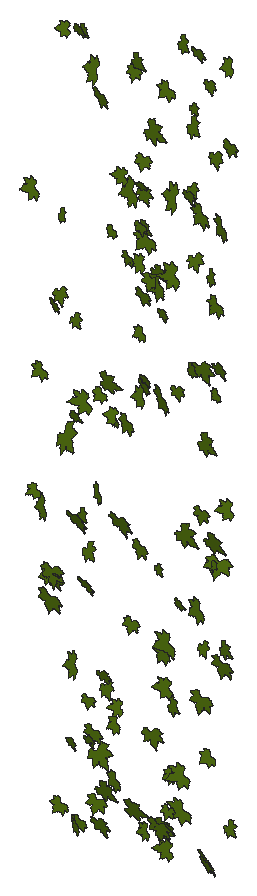
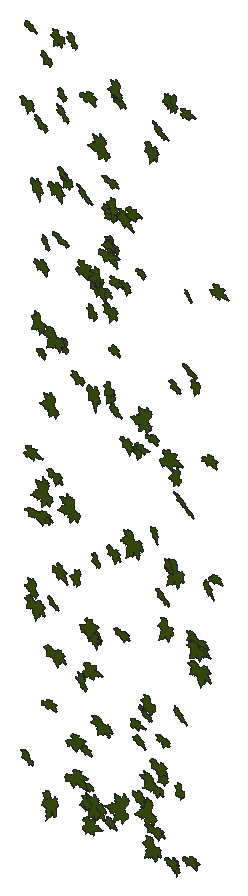
# SketchUp Ruby script. Lengths in inches.
U = 1.inch
M = Sketchup.active_model
def pt(a) = Geom::Point3d.new(a.map { |v| v * U })
def face(e, loops, mat)
  f = e.add_face(loops[0].map { |a| pt(a) })
  loops[1..].each { |l| e.add_face(l.map { |a| pt(a) }).erase! }
  f.material = f.back_material = mat if mat
  f
end
# faces: each face lists its corners as indices into pts; further lists are holes
def faces(e, pts, list, mat = nil) = list.each { |f| face(e, (f[0].is_a?(Array) ? f : [f]).map { |l| l.map { |i| pts[i] } }, mat) }
# xy, xz, yz: faces in a plane at the given z, y or x. An outline is a flat list of corners, or four numbers for a rectangle; further outlines are holes
def ring(l) = l.size == 4 ? [[l[0], l[1]], [l[2], l[1]], [l[2], l[3]], [l[0], l[3]]] : l.each_slice(2).to_a
def flat(e, list, mat, &to3) = list.each { |f| face(e, (f[0].is_a?(Array) ? f : [f]).map { |l| ring(l).map { |u, v| to3.(u, v) } }, mat) }
def xy(e, z, list, mat = nil) = flat(e, list, mat) { |x, y| [x, y, z] }
def xz(e, y, list, mat = nil) = flat(e, list, mat) { |x, z| [x, y, z] }
def yz(e, x, list, mat = nil) = flat(e, list, mat) { |y, z| [x, y, z] }
def lines(e, pts, list) = list.each { |a, b| e.add_line(pt(pts[a]), pt(pts[b])) }
# prism: a flat outline (further loops are holes) pulled along v
def prism(e, loops, v, mat = nil)
  f = face(e, loops, mat); d = Geom::Vector3d.new(v.map { |x| x * U })
  f.pushpull(f.normal.samedirection?(d) ? d.length : -d.length)
end
def box(e, o, s, mat = nil) = prism(e, [[o, [o[0] + s[0], o[1], o[2]], [o[0] + s[0], o[1] + s[1], o[2]], [o[0], o[1] + s[1], o[2]]]], [0, 0, s[2]], mat)
def at(x, y, z, deg = 0) = Geom::Transformation.translation(pt([x, y, z])) * Geom::Transformation.rotation(ORIGIN, Z_AXIS, deg.degrees)
def axes(o, x, y, z) = Geom::Transformation.new([*x, 0, *y, 0, *z, 0, *pt(o).to_a, 1])
def part(name) = M.definitions.add(name)
# library, detail: a bought-in or finely detailed component or shape, given as its bounding box
def library(name, o, s) = part(name).tap { |d| box(d.entities, o, s) }
def detail(e, o, s) = box(e.add_group.entities, o, s)
def put(e, d, t, mat = nil) = e.add_instance(d, t).tap { |i| i.material = mat if mat }
def group(e, t, mat = nil) = e.add_group.tap { |g| g.transformation = t; g.material = mat if mat }.entities
root = M.entities
M.materials.add("[Vegetation Blur 03]").color = [83, 114, 18]
c1 = part("ivy")
xy(c1.entities,0,[[0.782,0,0.786,0,0.787,0.005,0.789,0.009,0.821,0.072,0.875,0.147,1.001,0.272,1.073,0.331,1.137,0.363,1.178,0.379,1.223,0.384,1.272,0.383,1.311,0.374,1.36,0.355,1.399,0.334,1.491,0.285,1.541,0.244,1.583,0.199,1.617,0.15,1.64,0.128,1.662,0.115,1.717,0.105,1.745,0.093,1.784,0.054,1.819,0.057,1.854,0.064,1.882,0.075,1.896,0.074,1.91,0.071,1.937,0.063,1.964,0.053,1.99,0.038,2.016,0.015,2.034,0.002,2.04,0,2.038,0.003,2.036,0.007,2.033,0.038,2.036,0.068,2.045,0.1,2.055,0.116,2.064,0.123,2.077,0.129,2.088,0.129,2.106,0.132,2.118,0.13,2.179,0.132,2.207,0.133,2.225,0.133,2.242,0.138,2.22,0.162,2.207,0.186,2.206,0.213,2.212,0.236,2.228,0.262,2.247,0.274,2.298,0.283,2.355,0.294,2.37,0.296,2.376,0.295,2.377,0.3,2.377,0.303,2.385,0.329,2.411,0.37,2.426,0.392,2.449,0.407,2.511,0.426,2.561,0.444,2.619,0.466,2.589,0.469,2.561,0.476,2.501,0.5,2.449,0.516,2.424,0.523,2.401,0.535,2.377,0.556,2.372,0.568,2.36,0.575,2.268,0.586,2.225,0.592,2.207,0.599,2.194,0.61,2.143,0.65,2.13,0.664,2.122,0.682,2.123,0.7,2.13,0.719,2.148,0.75,2.17,0.781,2.195,0.807,2.221,0.828,2.284,0.874,2.291,0.88,2.288,0.887,2.276,0.9,2.267,0.916,2.265,0.933,2.273,0.967,2.292,1.002,2.313,1.03,2.334,1.054,2.348,1.067,2.358,1.074,2.363,1.076,2.362,1.081,2.35,1.094,2.347,1.11,2.35,1.143,2.359,1.18,2.385,1.254,2.415,1.324,2.448,1.393,2.45,1.4,2.446,1.398,2.44,1.394,2.427,1.383,2.402,1.36,2.376,1.339,2.345,1.324,2.305,1.309,2.282,1.303,2.273,1.306,2.245,1.294,2.212,1.287,2.187,1.291,2.163,1.301,2.142,1.316,2.134,1.327,2.124,1.325,2.09,1.292,2.053,1.259,2.014,1.234,1.973,1.215,1.954,1.21,1.931,1.208,1.909,1.212,1.893,1.22,1.879,1.233,1.872,1.248,1.867,1.281,1.864,1.319,1.821,1.258,1.773,1.197,1.726,1.141,1.698,1.121,1.679,1.116,1.666,1.117,1.647,1.122,1.632,1.129,1.62,1.141,1.617,1.154,1.617,1.219,1.621,1.254,1.623,1.268,1.623,1.281,1.618,1.314,1.606,1.346,1.603,1.375,1.607,1.403,1.603,1.467,1.599,1.499,1.605,1.525,1.614,1.552,1.629,1.577,1.635,1.589,1.629,1.587,1.618,1.582,1.596,1.566,1.581,1.556,1.568,1.552,1.557,1.55,1.545,1.553,1.531,1.562,1.522,1.572,1.504,1.591,1.486,1.611,1.474,1.631,1.457,1.666,1.455,1.684,1.457,1.698,1.452,1.715,1.444,1.728,1.424,1.754,1.419,1.772,1.423,1.786,1.434,1.819,1.444,1.848,1.446,1.855,1.44,1.861,1.43,1.867,1.386,1.904,1.349,1.948,1.326,1.973,1.31,1.995,1.288,2.048,1.284,2.153,1.287,2.254,1.284,2.255,1.282,2.253,1.278,2.247,1.274,2.237,1.266,2.216,1.226,2.125,1.208,2.076,1.184,2.033,1.155,1.984,1.135,1.942,1.111,1.899,1.083,1.861,1.053,1.85,1.059,1.83,1.061,1.809,1.056,1.79,1.049,1.767,1.04,1.749,1.018,1.733,0.994,1.726,0.942,1.734,0.95,1.6875,0.944,1.645,0.932,1.608,0.911,1.585,0.881,1.58,0.854,1.582,0.828,1.588,0.785,1.618,0.773,1.625,0.775,1.614,0.779,1.598,0.796,1.502,0.818,1.402,0.861,1.283,0.882,1.224,0.894,1.174,0.892,1.148,0.886,1.123,0.881,1.107,0.872,1.099,0.849,1.094,0.818,1.092,0.789,1.098,0.762,1.107,0.753,1.113,0.721,1.139,0.698,1.163,0.678,1.194,0.665,1.224,0.628,1.28,0.612,1.312,0.606,1.327,0.606,1.314,0.599,1.282,0.594,1.267,0.581,1.256,0.544,1.245,0.512,1.244,0.473,1.249,0.444,1.256,0.382,1.288,0.339,1.306,0.324,1.316,0.317,1.324,0.309,1.326,0.27,1.314,0.227,1.313,0.185,1.3125,0.152,1.317,0.122,1.328,0.092,1.345,0.073,1.353,0.079,1.338,0.092,1.308,0.117,1.249,0.13,1.215,0.139,1.164,0.147,1.148,0.157,1.136,0.163,1.122,0.174,1.086,0.177,1.067,0.182,1.054,0.186,1.043,0.191,1.038,0.211,1.028,0.237,1.005,0.25,0.974,0.253,0.96,0.25,0.944,0.242,0.914,0.243,0.906,0.249,0.902,0.26,0.894,0.289,0.88,0.307,0.873,0.322,0.862,0.364,0.799,0.403,0.738,0.431,0.709,0.439,0.691,0.441,0.678,0.4375,0.66,0.428,0.645,0.394,0.623,0.303,0.594,0.255,0.581,0.214,0.577,0.179,0.573,0.173,0.568,0.175,0.561,0.167,0.55,0.141,0.523,0.113,0.503,0.077,0.49,0.045,0.486,0.026,0.485,0.019,0.486,0.011,0.483,0,0.471,0.014,0.467,0.044,0.455,0.058,0.447,0.07,0.438,0.097,0.411,0.125,0.394,0.158,0.377,0.174,0.366,0.182,0.359,0.185,0.361,0.242,0.331,0.253,0.316,0.258,0.303,0.262,0.283,0.274,0.278,0.308,0.274,0.341,0.252,0.366,0.226,0.366,0.222,0.37,0.22,0.38,0.221,0.395,0.221,0.425,0.216,0.45,0.207,0.465,0.192,0.473,0.178,0.484,0.15,0.489,0.116,0.483,0.089,0.468,0.058,0.45,0.035,0.435,0.018,0.429,0.011,0.434,0.012,0.438,0.014,0.469,0.019,0.542,0.016,0.581,0.015,0.612,0.027,0.68,0.055,0.696,0.057,0.712,0.052,0.73,0.045,0.741,0.036,0.766,0.014]])
put(root,c1,axes([10.25,173.2,134.86],[0.22705,-0.11945,-0.35491],[-0.43835,-0.02,-0.18572],[-0.01818,-1.0093,0.04569]),"[Vegetation Blur 03]")
put(root,c1,axes([10.26,173.2,118.84],[0.22258,-0.06561,-0.19839],[-0.24493,-0.08915,-0.17839],[0.01076,-0.67235,0.04301]),"[Vegetation Blur 03]")
put(root,c1,axes([10.48,173.2,125.33],[0.3254,-0.08509,-0.21734],[-0.269,-0.05049,-0.26515],[-0.01633,-0.86378,0.03691]),"[Vegetation Blur 03]")
put(root,c1,axes([10.78,173.2,118.41],[0.27571,-0.25978,-0.33675],[-0.40528,0.18997,-0.24407],[-0.14812,-1.00337,0.04098]),"[Vegetation Blur 03]")
put(root,c1,axes([11.13,173.2,114.67],[0.1748,-0.10036,-0.26156],[-0.32362,-0.01023,-0.14344],[-0.01895,-0.75115,0.0369]),"[Vegetation Blur 03]")
put(root,c1,axes([10.51,173.2,113.55],[0.65346,-0.15996,-0.07236],[-0.08578,0.05992,-0.53686],[-0.0809,-1.3557,-0.01519]),"[Vegetation Blur 03]")
put(root,c1,axes([11.11,173.2,128.88],[0.3582,-0.18702,-0.03708],[-0.03384,0.10347,-0.29982],[-0.09581,-0.73577,-0.03274]),"[Vegetation Blur 03]")
put(root,c1,axes([10.59,173.2,114.79],[0.61675,-0.12461,0.11294],[0.13479,-0.08629,-0.50526],[-0.06818,-1.29784,0.02275]),"[Vegetation Blur 03]")
put(root,c1,axes([10.76,173.2,114.26],[0.44883,-0.14962,0.17944],[0.22549,0.05754,-0.36812],[-0.05276,-1.02686,-0.04677]),"[Vegetation Blur 03]")
put(root,c1,axes([11.51,173.2,102.9],[0.37574,-0.07096,-0.15978],[-0.19839,-0.07956,-0.3052],[-0.01253,-0.86822,0.04103]),"[Vegetation Blur 03]")
put(root,c1,axes([11.29,173.2,129.23],[0.32579,-0.0019,0.20222],[0.24053,-0.19974,-0.25841],[-0.05947,-0.81825,0.06261]),"[Vegetation Blur 03]")
put(root,c1,axes([11.61,173.2,133.17],[0.07732,0.04701,0.24249],[0.28519,-0.19481,-0.05463],[-0.0864,-0.60099,0.03668]),"[Vegetation Blur 03]")
put(root,c1,axes([12.29,173.2,143.72],[0.09099,-0.0894,-0.27257],[-0.33609,-0.07013,-0.07111],[0.02177,-0.70885,0.04141]),"[Vegetation Blur 03]")
put(root,c1,axes([11.42,173.2,121.39],[0.26041,0.16269,0.49935],[0.59768,-0.40532,-0.18684],[-0.15294,-1.30696,0.1201]),"[Vegetation Blur 03]")
put(root,c1,axes([12.69,173.2,110.82],[0.25932,-0.29593,-0.35358],[-0.43934,0.11655,-0.22996],[-0.12392,-1.03246,0.07539]),"[Vegetation Blur 03]")
put(root,c1,axes([12.05,173.2,106.03],[0.27088,-0.15261,0.15464],[0.19269,-0.01614,-0.22733],[-0.06536,-0.68006,-0.0293]),"[Vegetation Blur 03]")
put(root,c1,axes([12.46,173.2,102.22],[0.37274,-0.27698,-0.10257],[-0.11734,0.09274,-0.32343],[-0.14192,-0.80413,-0.00197]),"[Vegetation Blur 03]")
put(root,c1,axes([12.29,173.2,122.97],[0.1451,-0.1312,0.25798],[0.3214,0.00081,-0.12034],[-0.02623,-0.71573,-0.04743]),"[Vegetation Blur 03]")
put(root,c1,axes([12.26,173.2,128.03],[0.20968,0.01131,0.23173],[0.28004,-0.12895,-0.16779],[-0.0472,-0.71481,0.03394]),"[Vegetation Blur 03]")
put(root,c1,axes([13.33,173.2,124.72],[0.17219,-0.03701,-0.43547],[-0.53302,-0.07752,-0.13935],[0.03036,-1.15115,0.02338]),"[Vegetation Blur 03]")
put(root,c1,axes([12.58,173.2,102.29],[0.37414,-0.10141,-0.07585],[-0.09511,-0.0243,-0.3074],[-0.04493,-0.79294,0.01912]),"[Vegetation Blur 03]")
put(root,c1,axes([11.99,173.2,117.96],[0.55336,-0.2755,0.17895],[0.23761,0.14136,-0.45516],[-0.0977,-1.21665,-0.0934]),"[Vegetation Blur 03]")
put(root,c1,axes([12.51,173.2,143.37],[0.16816,-0.15089,0.24654],[0.3088,-0.00002,-0.1403],[-0.03567,-0.71145,-0.05229]),"[Vegetation Blur 03]")
put(root,c1,axes([12.74,173.2,117.9],[0.13772,-0.02232,0.26418],[0.31478,-0.16115,-0.11144],[-0.07624,-0.70573,0.01709]),"[Vegetation Blur 03]")
put(root,c1,axes([12.8,173.2,143.37],[0.14289,-0.07488,0.25812],[0.31299,-0.09737,-0.11985],[-0.0582,-0.70749,-0.01082]),"[Vegetation Blur 03]")
put(root,c1,axes([12.6875,173.2,114.76],[0.46892,-0.24319,0.11777],[0.16224,0.13537,-0.38629],[-0.09203,-1.00049,-0.08089]),"[Vegetation Blur 03]")
put(root,c1,axes([13.02,173.2,108.71],[0.35341,-0.05372,0.02619],[0.03014,-0.05475,-0.28854],[-0.02834,-0.72817,0.01976]),"[Vegetation Blur 03]")
put(root,c1,axes([13.05,173.2,106.5],[0.29444,-0.13699,0.14225],[0.1786,0.0132,-0.24425],[-0.05394,-0.70397,-0.03226]),"[Vegetation Blur 03]")
put(root,c1,axes([12.96,173.2,116.09],[0.20883,0.04815,0.31421],[0.37772,-0.20796,-0.1622],[-0.0781,-0.87697,0.05572]),"[Vegetation Blur 03]")
put(root,c1,axes([14.09,173.2,142.43],[0.1383,-0.27518,-0.42018],[-0.52123,0.14835,-0.12955],[-0.10615,-1.08693,0.0887]),"[Vegetation Blur 03]")
put(root,c1,axes([13.23,173.2,107.3],[0.4987,-0.12613,-0.04723],[-0.0598,-0.02572,-0.40975],[-0.05942,-1.03278,0.01597]),"[Vegetation Blur 03]")
put(root,c1,axes([13.88,173.2,120.12],[0.31941,-0.24553,-0.21108],[-0.24847,0.1507,-0.27802],[-0.13923,-0.8322,0.01193]),"[Vegetation Blur 03]")
put(root,c1,axes([13.45,173.2,103.7],[0.48615,-0.06506,-0.03255],[-0.04363,-0.12709,-0.39413],[-0.0262,-0.99568,0.05243]),"[Vegetation Blur 03]")
put(root,c1,axes([13.94,173.2,125.18],[0.29981,-0.06525,-0.13535],[-0.1686,-0.07812,-0.24283],[-0.00912,-0.70071,0.03968]),"[Vegetation Blur 03]")
put(root,c1,axes([13.67,173.2,140.84],[0.50217,-0.23211,-0.02067],[-0.01614,0.08923,-0.41886],[-0.11447,-1.03084,-0.03161]),"[Vegetation Blur 03]")
put(root,c1,axes([13.21,173.2,105.65],[0.43574,0.04341,0.40329],[0.4922,-0.17124,-0.35133],[-0.04861,-1.34487,0.05775]),"[Vegetation Blur 03]")
put(root,c1,axes([13.42,173.2,102.36],[0.49317,-0.18476,0.20262],[0.2548,0.0498,-0.40595],[-0.06909,-1.1351,-0.05079]),"[Vegetation Blur 03]")
put(root,c1,axes([13.78,173.2,110.15],[0.36419,-0.14328,0.1768],[0.2225,0.04791,-0.29916],[-0.04769,-0.87068,-0.04556]),"[Vegetation Blur 03]")
put(root,c1,axes([13.74,173.2,103.85],[0.29611,-0.16504,0.41768],[0.51687,0.01316,-0.24325],[-0.03458,-1.21665,-0.05929]),"[Vegetation Blur 03]")
put(root,c1,axes([14.02,173.2,109.44],[0.29238,-0.00543,0.2431],[0.28843,-0.20948,-0.23179],[-0.07444,-0.83296,0.05671]),"[Vegetation Blur 03]")
put(root,c1,axes([15.16,173.2,124.375],[0.04403,-0.12753,-0.27738],[-0.34532,-0.03734,-0.03381],[0.01033,-0.70424,0.05202]),"[Vegetation Blur 03]")
put(root,c1,axes([14.64,173.2,133.94],[0.27643,-0.11245,-0.0959],[-0.1208,-0.01738,-0.22873],[-0.04691,-0.61786,0.02389]),"[Vegetation Blur 03]")
put(root,c1,axes([14.13,173.2,125.11],[0.08822,-0.12322,0.46198],[0.56917,0.00464,-0.0722],[-0.00698,-1.17889,-0.04857]),"[Vegetation Blur 03]")
put(root,c1,axes([14.81,173.2,105.4],[0.34978,-0.17504,-0.23097],[-0.28247,0.06704,-0.29293],[-0.08681,-0.92345,0.02252]),"[Vegetation Blur 03]")
put(root,c1,axes([14.97,173.2,108.375],[0.28202,-0.18926,-0.22565],[-0.28437,-0.00619,-0.23592],[-0.06351,-0.81269,0.05435]),"[Vegetation Blur 03]")
put(root,c1,axes([14.73,173.2,123.98],[0.28723,-0.15203,-0.02555],[-0.02588,0.0511,-0.24162],[-0.07595,-0.59236,-0.01429]),"[Vegetation Blur 03]")
put(root,c1,axes([15.34,173.2,109.22],[0.11929,-0.10597,-0.2818],[-0.34889,-0.06251,-0.09467],[0.01224,-0.74914,0.04776]),"[Vegetation Blur 03]")
put(root,c1,axes([15.65,173.2,137.16],[0.05825,-0.05857,-0.32384],[-0.39732,-0.0501,-0.04618],[0.02002,-0.82377,0.02584]),"[Vegetation Blur 03]")
put(root,c1,axes([14.51,173.2,118.8],[0.63866,-0.23189,0.12864],[0.16822,0.10928,-0.52532],[-0.09614,-1.34925,-0.06466]),"[Vegetation Blur 03]")
put(root,c1,axes([15.37,173.2,124.36],[0.44792,-0.20906,-0.13241],[-0.16237,0.03502,-0.37455],[-0.10139,-0.9797,0.01487]),"[Vegetation Blur 03]")
put(root,c1,axes([15.47,173.2,132.87],[0.35103,-0.1488,-0.07514],[-0.0909,0.03087,-0.29249],[-0.07377,-0.74614,0.00288]),"[Vegetation Blur 03]")
put(root,c1,axes([15.96,173.2,136.93],[0.36429,-0.26691,-0.39719],[-0.49048,0.09297,-0.30946],[-0.1145,-1.24751,0.06192]),"[Vegetation Blur 03]")
put(root,c1,axes([15.54,173.2,113.7],[0.40879,-0.06868,-0.00639],[-0.01176,-0.09983,-0.33231],[-0.0322,-0.83542,0.04024]),"[Vegetation Blur 03]")
put(root,c1,axes([15.76,173.2,142.72],[0.38042,-0.08348,0.02066],[0.01844,-0.12918,-0.30833],[-0.04412,-0.77385,0.04924]),"[Vegetation Blur 03]")
put(root,c1,axes([16.62,173.2,133.02],[0.14335,-0.13764,-0.29117],[-0.36286,-0.03379,-0.11648],[-0.00945,-0.79049,0.05568]),"[Vegetation Blur 03]")
put(root,c1,axes([16.59,173.2,126.09],[0.18991,-0.19032,-0.31472],[-0.38839,0.08836,-0.16451],[-0.08006,-0.88012,0.05154]),"[Vegetation Blur 03]")
put(root,c1,axes([15.59,173.2,103.26],[0.11966,-0.19885,0.48664],[0.60405,0.04067,-0.09632],[0.00062,-1.25082,-0.0805]),"[Vegetation Blur 03]")
put(root,c1,axes([16.45,173.2,129.25],[0.22039,-0.10268,-0.20891],[-0.2592,-0.01,-0.18136],[-0.02883,-0.69502,0.03347]),"[Vegetation Blur 03]")
put(root,c1,axes([15.89,173.2,142.71],[0.15082,-0.08194,0.36497],[0.44384,-0.11913,-0.12637],[-0.06768,-0.96384,-0.01541]),"[Vegetation Blur 03]")
put(root,c1,axes([16.07,173.2,117.99],[0.46442,-0.17928,-0.04706],[-0.05947,-0.00913,-0.38545],[-0.0859,-0.96299,0.01241]),"[Vegetation Blur 03]")
put(root,c1,axes([16.07,173.2,134.55],[0.32611,-0.0735,0.11387],[0.13621,-0.07341,-0.2673],[-0.04678,-0.72621,0.01549]),"[Vegetation Blur 03]")
put(root,c1,axes([16.78,173.2,103.31],[0.2031,-0.14404,-0.26055],[-0.32267,0.0347,-0.17055],[-0.052,-0.77785,0.04064]),"[Vegetation Blur 03]")
put(root,c1,axes([16.08,173.2,136.54],[0.28631,-0.17737,0.19402],[0.25002,0.08801,-0.2331],[-0.03783,-0.76071,-0.07221]),"[Vegetation Blur 03]")
put(root,c1,axes([16.17,173.2,131.22],[0.46399,-0.15608,-0.0301],[-0.03246,0.06122,-0.3832],[-0.07784,-0.95586,-0.01963]),"[Vegetation Blur 03]")
put(root,c1,axes([16.22,173.2,138.21],[0.40348,-0.0468,0.02113],[0.02171,-0.14086,-0.32526],[-0.02676,-0.81998,0.05467]),"[Vegetation Blur 03]")
put(root,c1,axes([16.51,173.2,134.51],[0.49046,-0.12487,-0.25125],[-0.31171,-0.05916,-0.40067],[-0.03597,-1.19015,0.04628]),"[Vegetation Blur 03]")
put(root,c1,axes([16.28,173.2,126.4],[0.3929,-0.21833,0.06927],[0.09371,0.04854,-0.33],[-0.09838,-0.82573,-0.03771]),"[Vegetation Blur 03]")
put(root,c1,axes([16.14,173.2,136.21],[0.36838,-0.06003,0.20905],[0.25298,-0.09287,-0.30112],[-0.04965,-0.91861,0.01678]),"[Vegetation Blur 03]")
put(root,c1,axes([16.36,173.2,126.58],[0.28308,-0.16005,0.12566],[0.16212,0.03888,-0.23548],[-0.05892,-0.66197,-0.04421]),"[Vegetation Blur 03]")
put(root,c1,axes([16.29,173.2,134.23],[0.16779,-0.0883,0.30239],[0.37001,-0.06611,-0.13979],[-0.04708,-0.83437,-0.02093]),"[Vegetation Blur 03]")
put(root,c1,axes([16.64,173.2,132.12],[0.43256,-0.06671,-0.01604],[-0.02325,-0.10108,-0.35159],[-0.02994,-0.88528,0.04135]),"[Vegetation Blur 03]")
put(root,c1,axes([16.4375,173.2,108.09],[0.51003,-0.05161,0.17077],[0.20792,-0.06034,-0.4165],[-0.03431,-1.13281,0.01441]),"[Vegetation Blur 03]")
put(root,c1,axes([17.36,173.2,132.52],[0.43677,-0.25618,-0.34823],[-0.42807,0.08886,-0.36791],[-0.11962,-1.25334,0.04509]),"[Vegetation Blur 03]")
put(root,c1,axes([16.61,173.2,139.19],[0.18628,-0.03587,0.49266],[0.60208,-0.08964,-0.15266],[-0.04677,-1.29689,-0.00307]),"[Vegetation Blur 03]")
put(root,c1,axes([16.98,173.2,132.26],[0.26264,-0.10696,0.28896],[0.35555,-0.0243,-0.21667],[-0.0405,-0.90682,-0.02828]),"[Vegetation Blur 03]")
put(root,c1,axes([16.84,173.2,103.66],[0.62439,-0.15847,0.04406],[0.05688,0.04229,-0.51297],[-0.0749,-1.28898,-0.02225]),"[Vegetation Blur 03]")
put(root,c1,axes([17.23,173.2,116.77],[0.18692,-0.08145,0.20202],[0.24238,-0.1034,-0.15594],[-0.06396,-0.62987,-0.00053]),"[Vegetation Blur 03]")
put(root,c1,axes([17.35,173.2,126.54],[0.55558,-0.31709,-0.23093],[-0.26347,0.22092,-0.46992],[-0.18545,-1.26384,-0.0242]),"[Vegetation Blur 03]")
put(root,c1,axes([18.2,173.2,111.32],[0.10909,-0.05884,-0.38294],[-0.46937,-0.06819,-0.08742],[0.02587,-0.98895,0.02881]),"[Vegetation Blur 03]")
put(root,c1,axes([18.27,173.2,102.81],[0.07011,-0.04175,-0.39035],[-0.47768,-0.07166,-0.05594],[0.03155,-0.99215,0.02047]),"[Vegetation Blur 03]")
put(root,c1,axes([17.45,173.2,113.06],[0.4568,-0.18649,-0.14633],[-0.18134,0.01163,-0.3794],[-0.08646,-1.00976,0.02265]),"[Vegetation Blur 03]")
put(root,c1,axes([17.99,173.2,113.83],[0.34831,-0.13161,-0.42418],[-0.52189,0.01831,-0.28634],[-0.04303,-1.28736,0.03929]),"[Vegetation Blur 03]")
put(root,c1,axes([17.4,173.2,130.4],[0.29752,-0.1463,0.14185],[0.17418,-0.03541,-0.24908],[-0.07018,-0.70816,-0.01685]),"[Vegetation Blur 03]")
put(root,c1,axes([17.25,173.2,102.9],[0.12855,-0.09811,0.43066],[0.52964,-0.00555,-0.1055],[-0.01392,-1.1176,-0.03728]),"[Vegetation Blur 03]")
put(root,c1,axes([17.85,173.2,142.65],[0.37323,-0.08724,-0.21133],[-0.2619,-0.06711,-0.30372],[-0.01607,-0.93236,0.04164]),"[Vegetation Blur 03]")
put(root,c1,axes([18.2,173.2,106.68],[0.22279,-0.12525,-0.19809],[-0.24846,-0.03124,-0.18302],[-0.02974,-0.67725,0.04508]),"[Vegetation Blur 03]")
put(root,c1,axes([17.78,173.2,104.61],[0.33968,-0.06301,-0.00772],[-0.01455,-0.11855,-0.2742],[-0.02856,-0.68915,0.04788]),"[Vegetation Blur 03]")
put(root,c1,axes([18.54,173.2,133.27],[0.22309,-0.1604,-0.43567],[-0.53899,-0.01598,-0.18291],[-0.02282,-1.19045,0.06116]),"[Vegetation Blur 03]")
put(root,c1,axes([18.73,173.2,137.38],[0.14321,-0.30149,-0.44399],[-0.54717,0.20081,-0.13901],[-0.13425,-1.14006,0.09293]),"[Vegetation Blur 03]")
put(root,c1,axes([17.74,173.2,103.37],[0.20518,-0.11933,0.20995],[0.26085,-0.0065,-0.17038],[-0.03866,-0.67709,-0.03537]),"[Vegetation Blur 03]")
put(root,c1,axes([18.04,173.2,109.59],[0.06873,0.01711,0.34805],[0.41669,-0.19262,-0.05332],[-0.09114,-0.86777,0.0187]),"[Vegetation Blur 03]")
put(root,c1,axes([18.63,173.2,105.28],[0.4097,-0.04709,-0.34938],[-0.42867,-0.05903,-0.33358],[0.00494,-1.21793,0.02968]),"[Vegetation Blur 03]")
put(root,c1,axes([18.84,173.2,107.16],[0.31711,-0.08877,-0.37028],[-0.45541,-0.10498,-0.25583],[0.01733,-1.13422,0.05266]),"[Vegetation Blur 03]")
put(root,c1,axes([18.17,173.2,126.63],[0.33984,-0.05336,0.11192],[0.13528,-0.05673,-0.27786],[-0.03432,-0.75199,0.01302]),"[Vegetation Blur 03]")
put(root,c1,axes([18.53,173.2,115.22],[0.06463,-0.12992,0.26421],[0.32679,-0.06667,-0.0584],[-0.04465,-0.67604,-0.04502]),"[Vegetation Blur 03]")
put(root,c1,axes([18.61,173.2,144.58],[0.1212,0.00874,0.32904],[0.39357,-0.19062,-0.09576],[-0.08752,-0.84508,0.025]),"[Vegetation Blur 03]")
put(root,c1,axes([18.37,173.2,118.82],[0.30964,-0.0676,0.45983],[0.56279,-0.06237,-0.25387],[-0.0424,-1.3215,-0.01154]),"[Vegetation Blur 03]")
put(root,c1,axes([18.89,173.2,137.17],[0.34101,-0.13421,0.11002],[0.1371,0.00224,-0.28262],[-0.06025,-0.75456,-0.02041]),"[Vegetation Blur 03]")
put(root,c1,axes([19.22,173.2,127.7],[0.0683,-0.05119,0.27634],[0.33407,-0.11649,-0.05839],[-0.06049,-0.70118,-0.01047]),"[Vegetation Blur 03]")
put(root,c1,axes([19.11,173.2,137.29],[0.21707,0.00977,0.22202],[0.26718,-0.14285,-0.17301],[-0.05136,-0.70178,0.03831]),"[Vegetation Blur 03]")
put(root,c1,axes([19.1,173.2,140.37],[0.13518,0.07282,0.36034],[0.43243,-0.22734,-0.10083],[-0.09589,-0.9226,0.05329]),"[Vegetation Blur 03]")
put(root,c1,axes([19.26,173.2,141.61],[0.18338,-0.0476,0.19783],[0.23906,-0.08339,-0.15076],[-0.04624,-0.61987,0.00509]),"[Vegetation Blur 03]")
put(root,c1,axes([19.75,173.2,116.17],[0.36665,-0.19895,-0.32997],[-0.4044,0.08632,-0.30749],[-0.09631,-1.11984,0.03492]),"[Vegetation Blur 03]")
put(root,c1,axes([19.15,173.2,133.73],[0.33502,0.02499,0.20079],[0.2423,-0.1873,-0.26561],[-0.04435,-0.83458,0.06562]),"[Vegetation Blur 03]")
put(root,c1,axes([19.36,173.2,144.86],[0.38814,-0.14356,0.10109],[0.12917,0.04667,-0.31993],[-0.05936,-0.83711,-0.03517]),"[Vegetation Blur 03]")
put(root,c1,axes([19.74,173.2,136.94],[0.49987,-0.22483,-0.22694],[-0.27931,0.04426,-0.41667],[-0.10606,-1.17624,0.0277]),"[Vegetation Blur 03]")
put(root,c1,axes([19.46,173.2,111.29],[0.58789,-0.11281,-0.04556],[-0.05859,-0.05769,-0.48112],[-0.05185,-1.21383,0.0271]),"[Vegetation Blur 03]")
put(root,c1,axes([19.59,173.2,120.92],[0.43658,-0.10423,0.00392],[0.00224,-0.04583,-0.35826],[-0.05083,-0.89729,0.01784]),"[Vegetation Blur 03]")
put(root,c1,axes([19.29,173.2,128.21],[0.52256,-0.08904,0.24501],[0.30058,-0.01277,-0.42774],[-0.04062,-1.24009,-0.01319]),"[Vegetation Blur 03]")
put(root,c1,axes([19.76,173.2,113.52],[0.23663,-0.00308,0.21961],[0.25991,-0.18831,-0.18695],[-0.06967,-0.71292,0.04843]),"[Vegetation Blur 03]")
put(root,c1,axes([20.35,173.2,108.46],[0.296,-0.08214,-0.20649],[-0.25613,-0.08908,-0.23898],[-0.00188,-0.79632,0.04803]),"[Vegetation Blur 03]")
put(root,c1,axes([19.9,173.2,102.66],[0.4103,-0.202,-0.00421],[0.00893,0.12198,-0.34084],[-0.09789,-0.83552,-0.04874]),"[Vegetation Blur 03]")
put(root,c1,axes([19.75,173.2,103.04],[0.61856,-0.3329,-0.06965],[-0.05285,0.26763,-0.51381],[-0.1751,-1.25675,-0.09097]),"[Vegetation Blur 03]")
put(root,c1,axes([19.75,173.2,123.99],[0.19561,-0.07372,0.44835],[0.54629,-0.12238,-0.16192],[-0.06809,-1.19373,-0.01109]),"[Vegetation Blur 03]")
put(root,c1,axes([20.15,173.2,143.36],[0.32177,-0.10077,0.13804],[0.16444,-0.08743,-0.26534],[-0.06299,-0.74292,0.0125]),"[Vegetation Blur 03]")
put(root,c1,axes([20.27,173.2,118.22],[0.28684,-0.06236,0.1063],[0.12625,-0.08285,-0.23456],[-0.04409,-0.64295,0.01992]),"[Vegetation Blur 03]")
put(root,c1,axes([20.32,173.2,132.93],[0.07908,0.01608,0.29029],[0.3424,-0.20709,-0.06032],[-0.09663,-0.72064,0.02381]),"[Vegetation Blur 03]")
put(root,c1,axes([20.79,173.2,127.49],[0.2496,-0.10992,-0.13236],[-0.16418,0.00788,-0.20725],[-0.04691,-0.61248,0.02109]),"[Vegetation Blur 03]")
put(root,c1,axes([20.66,173.2,132.38],[0.42696,-0.16855,-0.18226],[-0.22665,-0.00186,-0.3534],[-0.07216,-0.99152,0.03164]),"[Vegetation Blur 03]")
put(root,c1,axes([20.35,173.2,118.63],[0.56687,0.06013,-0.01984],[-0.01943,-0.18427,-0.45761],[0.03267,-1.15295,0.0721]),"[Vegetation Blur 03]")
put(root,c1,axes([20.1,173.2,119.1],[0.31154,-0.18802,0.42817],[0.53015,-0.00865,-0.25753],[-0.0503,-1.25557,-0.06234]),"[Vegetation Blur 03]")
put(root,c1,axes([20.42,173.2,139.62],[0.34903,-0.06561,0.18456],[0.21828,-0.15404,-0.28357],[-0.06714,-0.84183,0.0375]),"[Vegetation Blur 03]")
put(root,c1,axes([20.97,173.2,136.71],[0.46455,-0.28541,-0.24702],[-0.29064,0.17394,-0.39567],[-0.16241,-1.12761,0.00149]),"[Vegetation Blur 03]")
put(root,c1,axes([20.54,173.2,128.62],[0.36896,-0.184,0.21842],[0.27276,0.00042,-0.30684],[-0.07226,-0.93795,-0.04299]),"[Vegetation Blur 03]")
put(root,c1,axes([20.67,173.2,113.57],[0.60359,-0.16861,-0.0634],[-0.07511,0.04962,-0.497],[-0.08431,-1.25133,-0.01117]),"[Vegetation Blur 03]")
put(root,c1,axes([21.75,173.2,121.94],[0.1638,-0.10041,-0.33523],[-0.41333,-0.07495,-0.13099],[0.01603,-0.90688,0.04794]),"[Vegetation Blur 03]")
put(root,c1,axes([21.04,173.2,113.66],[0.12722,-0.05638,0.35512],[0.42991,-0.13892,-0.10606],[-0.07252,-0.92248,-0.00573]),"[Vegetation Blur 03]")
put(root,c1,axes([21.8,173.2,145.1875],[0.2034,-0.19719,-0.25526],[-0.32297,-0.00076,-0.17132],[-0.05192,-0.76775,0.06573]),"[Vegetation Blur 03]")
put(root,c1,axes([21.33,173.2,140.77],[0.4277,-0.13208,-0.01923],[-0.02433,-0.00684,-0.35292],[-0.0639,-0.88143,0.00562]),"[Vegetation Blur 03]")
put(root,c1,axes([21.26,173.2,104.45],[0.18478,0.02807,0.2907],[0.35178,-0.14758,-0.1467],[-0.05752,-0.81244,0.03669]),"[Vegetation Blur 03]")
